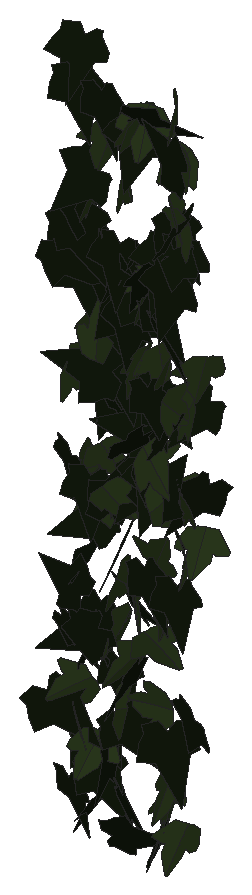
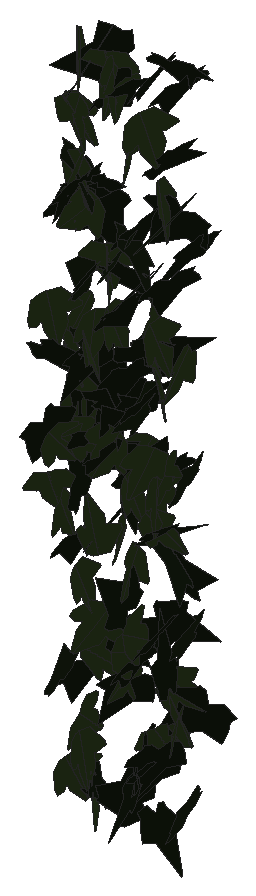
# SketchUp Ruby script. Lengths in inches.
U = 1.inch
M = Sketchup.active_model
def pt(a) = Geom::Point3d.new(a.map { |v| v * U })
def face(e, loops, mat)
  f = e.add_face(loops[0].map { |a| pt(a) })
  loops[1..].each { |l| e.add_face(l.map { |a| pt(a) }).erase! }
  f.material = f.back_material = mat if mat
  f
end
# faces: each face lists its corners as indices into pts; further lists are holes
def faces(e, pts, list, mat = nil) = list.each { |f| face(e, (f[0].is_a?(Array) ? f : [f]).map { |l| l.map { |i| pts[i] } }, mat) }
# xy, xz, yz: faces in a plane at the given z, y or x. An outline is a flat list of corners, or four numbers for a rectangle; further outlines are holes
def ring(l) = l.size == 4 ? [[l[0], l[1]], [l[2], l[1]], [l[2], l[3]], [l[0], l[3]]] : l.each_slice(2).to_a
def flat(e, list, mat, &to3) = list.each { |f| face(e, (f[0].is_a?(Array) ? f : [f]).map { |l| ring(l).map { |u, v| to3.(u, v) } }, mat) }
def xy(e, z, list, mat = nil) = flat(e, list, mat) { |x, y| [x, y, z] }
def xz(e, y, list, mat = nil) = flat(e, list, mat) { |x, z| [x, y, z] }
def yz(e, x, list, mat = nil) = flat(e, list, mat) { |y, z| [x, y, z] }
def lines(e, pts, list) = list.each { |a, b| e.add_line(pt(pts[a]), pt(pts[b])) }
# prism: a flat outline (further loops are holes) pulled along v
def prism(e, loops, v, mat = nil)
  f = face(e, loops, mat); d = Geom::Vector3d.new(v.map { |x| x * U })
  f.pushpull(f.normal.samedirection?(d) ? d.length : -d.length)
end
def box(e, o, s, mat = nil) = prism(e, [[o, [o[0] + s[0], o[1], o[2]], [o[0] + s[0], o[1] + s[1], o[2]], [o[0], o[1] + s[1], o[2]]]], [0, 0, s[2]], mat)
def at(x, y, z, deg = 0) = Geom::Transformation.translation(pt([x, y, z])) * Geom::Transformation.rotation(ORIGIN, Z_AXIS, deg.degrees)
def axes(o, x, y, z) = Geom::Transformation.new([*x, 0, *y, 0, *z, 0, *pt(o).to_a, 1])
def part(name) = M.definitions.add(name)
# library, detail: a bought-in or finely detailed component or shape, given as its bounding box
def library(name, o, s) = part(name).tap { |d| box(d.entities, o, s) }
def detail(e, o, s) = box(e.add_group.entities, o, s)
def put(e, d, t, mat = nil) = e.add_instance(d, t).tap { |i| i.material = mat if mat }
def group(e, t, mat = nil) = e.add_group.tap { |g| g.transformation = t; g.material = mat if mat }.entities
root = M.entities
M.materials.add("efeu1").color = [18, 25, 13]
M.materials.add("efeu2").color = [43, 57, 29]
c1 = part("ivyleaf_9")
p = [[1.54,2.16,1.25],[1.36,2.04,1.19],[-0.21,0.99,0.68],[-0.71,1.11,0.82],[-0.85,0.86,0.67],[-0.8,0.17,0.21],
  [-0.9,-0.01,0.1],[-0.67,-0.16,-0.02],[-0.08,-0.08,-0.05],[-0.03,-0.6,-0.4],[0.65,-0.88,-0.66],[0.83,-0.6,-0.49],
  [1.29,-0.42,-0.43],[1.8125,-0.07,-0.26],[1.21,0.44,0.15]]
faces(c1.entities,p,[[0,1,2,3,4,5,6,7,8,9,10,11,12,13,14]],"efeu1")
c2 = part("ivyleaf_10")
p = [[0,0.5,-0.03],[-0.0625,2.02,-0.43],[-0.19,2.01,-0.46],[-0.54,1.05,-0.29],[-0.52,0.625,-0.18],[-0.83,0.76,-0.28],
  [-1.16,0.64,-0.33],[-1.15,0.33,-0.24],[-0.77,-0.39,0.02],[-0.3,-0.51,0.16],[0.04,-0.48,0.23],[-0.02,2.01,-0.4375],
  [-0.06,2.01,-0.43],[0.04,-0.49,0.23],[0.67,-0.49,0.14],[1.38,0.36,-0.2],[1.375,0.51,-0.24],[0.81,0.65,-0.19],
  [0.62,0.59,-0.15],[0.6,1.09,-0.28],[0.5,1.23,-0.31]]
faces(c2.entities,p,[[0,1,2,3,4,5,6,7,8,9,10],[11,12,0,13,14,15,16,17,18,19,20]],"efeu2")
put(root,c1,axes([551.875,130.74,243.39],[-0.73548,-0.58268,-0.39107],[0.45946,0.02837,-0.90635],[0.53043,-0.8325,0.24283]))
put(root,c2,axes([551.63,130.18,211.08],[0.71363,-0.41325,-0.37001],[0.32522,-0.1767,0.82459],[-0.44935,-0.78419,0.00919]))
put(root,c1,axes([551.56,130.29,223.09],[0.17606,-0.69879,0.57439],[0.16825,-0.54966,-0.72027],[0.88877,0.24248,0.02257]))
put(root,c1,axes([551.46,128.98,212.17],[-0.08461,-0.32364,-1.03938],[0.63838,0.8297,-0.31032],[0.88178,-0.63173,0.12492]))
put(root,c1,axes([551.58,130.1875,207.4],[0.4557,-0.79853,0.24374],[0.10831,-0.21879,-0.9193],[0.82784,0.46819,-0.0139]))
put(root,c1,axes([551.75,129.03,234.1],[0.54072,-0.53779,-0.74074],[-0.22529,0.75567,-0.71309],[0.88722,0.51965,0.27038]))
put(root,c2,axes([552.82,129.55,212.97],[-0.44073,-0.23806,0.79955],[-0.61172,-0.52263,-0.49281],[0.56723,-0.74859,0.08978]))
put(root,c1,axes([551.875,129.42,215.66],[0.72537,-0.54547,-0.21984],[-0.11834,0.20656,-0.90298],[0.57608,0.72927,0.09133]))
put(root,c2,axes([552.93,130.6875,221.07],[-0.56763,0.02035,0.73262],[-0.65899,-0.41973,-0.49892],[0.32076,-0.8263,0.27148]))
put(root,c1,axes([552.2,130.6,213.66],[0.04903,0.69244,0.79719],[-0.13822,-0.78697,0.69207],[1.04684,-0.13634,0.05403]))
put(root,c1,axes([552.09,129.99,241.96],[0.10131,-0.9926,-0.20243],[0.02815,0.20612,-0.9966],[1.01264,0.09357,0.04796]))
put(root,c1,axes([553.18,128.72,217.72],[-0.19941,0.13422,0.89928],[-0.69386,0.57251,-0.23931],[-0.5876,-0.72159,-0.02259]))
put(root,c2,axes([552.375,130.49,223.46],[-0.04635,0.50692,-0.77285],[0.02045,-0.77307,-0.50829],[-0.92404,-0.04253,0.02752]))
put(root,c1,axes([552.99,129.21,218.8],[-0.20039,0.78529,0.56916],[-0.1994,0.53541,-0.80893],[-0.94914,-0.27828,0.04978]))
put(root,c2,axes([552.58,130.93,230.2],[0.06623,-0.95926,0.25328],[0.02269,-0.25231,-0.96153],[0.99187,0.06983,0.00508]))
put(root,c2,axes([552.44,129.15,228.34],[0.18841,-0.77312,-0.71532],[0.22398,0.73946,-0.74022],[1.02919,-0.0194,0.29204]))
put(root,c1,axes([552.24,130.46,232.69],[-0.04103,-0.92797,-0.29273],[0.03155,0.29157,-0.92871],[0.97254,-0.04861,0.01778]))
put(root,c2,axes([552.625,129.37,211.4],[-0.52676,0.73649,0.16397],[-0.11717,0.1177,-0.90509],[-0.74537,-0.53899,0.02641]))
put(root,c2,axes([552.61,130.81,228.21],[0.62375,-0.71751,-0.12292],[-0.04467,0.12384,-0.94956],[0.72659,0.62357,0.04714]))
put(root,c1,axes([552.95,130.4,206.96],[-0.39182,0.78825,-0.28221],[0.08901,-0.27061,-0.87941],[-0.83251,-0.39992,0.0388]))
put(root,c1,axes([552.98,130.84,220.37],[-0.65916,-0.26857,0.61132],[-0.35575,-0.58569,-0.64089],[0.56506,-0.68203,0.30963]))
put(root,c1,axes([552.19,129.89,235.78],[0.66785,-0.57956,-0.4415],[-0.13878,0.48676,-0.8489],[0.71523,0.63561,0.24754]))
put(root,c2,axes([552.81,130.49,222.6],[0.03199,-0.9257,-0.29655],[0.03115,0.29753,-0.92542],[0.97154,0.02094,0.03944]))
put(root,c2,axes([552.92,130.12,236.52],[0.37549,-0.93857,-0.20251],[-0.04385,0.20046,-1.01035],[0.95916,0.37659,0.03309]))
put(root,c1,axes([552.57,131.05,215.91],[0.20574,-0.92635,0.10949],[0.01826,-0.1081,-0.94891],[0.93262,0.20648,-0.00558]))
put(root,c1,axes([552.41,129.49,235.5],[-0.32673,-0.47618,-0.97385],[0.80772,0.57143,-0.55041],[0.723,-0.85358,0.17481]))
put(root,c1,axes([553.56,129.47,215.78],[-0.15472,-0.05646,-0.93104],[-0.37886,-0.8586,0.11503],[-0.85235,0.39189,0.11788]))
put(root,c1,axes([553.16,129.88,237.75],[-0.46724,-0.678,0.58718],[-0.2175,-0.55666,-0.81584],[0.87015,-0.5032,0.11137]))
put(root,c1,axes([552.96,130.32,209.98],[-0.04159,-0.76272,-0.61098],[-0.00593,0.61172,-0.76324],[0.97725,-0.02874,-0.03064]))
put(root,c2,axes([553.23,130.56,223.95],[-0.59059,-0.61552,-0.4088],[0.32802,0.25054,-0.85112],[0.66211,-0.67316,0.05702]))
put(root,c1,axes([553.15,131.18,226.97],[-0.14366,-0.92937,0.24009],[-0.0217,-0.23956,-0.94029],[0.95963,-0.14455,0.01468]))
put(root,c1,axes([554.01,129.77,228.35],[-0.52949,-0.5655,-0.666],[-0.2161,-0.66979,0.74053],[-0.84655,0.52468,0.22752]))
put(root,c2,axes([553.51,129.51,210.26],[0.6923,0.48876,-0.3775],[-0.29893,-0.23103,-0.84731],[-0.54041,0.75393,-0.01491]))
put(root,c2,axes([553.63,130.4375,239.68],[-0.45807,-0.87367,0.30003],[-0.05476,-0.30863,-0.98229],[0.92213,-0.45232,0.09071]))
put(root,c1,axes([553.6,131.15,229.36],[-0.66621,-0.65807,0.06911],[-0.04349,-0.05431,-0.93639],[0.66025,-0.66758,0.00805]))
put(root,c1,axes([553.26,129.51,222.96],[-0.08448,-0.91933,-0.11123],[-0.00032,0.11172,-0.92315],[0.92604,-0.08383,-0.01046]))
put(root,c1,axes([553.28,129.9375,209],[0.16461,-0.78141,-0.53609],[-0.01765,0.54149,-0.7947],[0.94746,0.14585,0.07834]))
put(root,c1,axes([553.11,130.89,226.72],[0.71599,-0.66448,0.00847],[0.00634,-0.00562,-0.97682],[0.66451,0.71602,0.0002]))
put(root,c2,axes([553.9,130.97,222.57],[0.16534,-0.90004,0.23776],[0.04672,-0.23316,-0.9151],[0.92974,0.17178,0.0037]))
put(root,c2,axes([554.07,128.74,229.93],[0.06984,0.83129,-0.62397],[-0.08929,0.62786,0.82649],[1.03558,-0.00193,0.11334]))
put(root,c2,axes([553.76,131.11,215.55],[0.19819,-0.45252,0.84638],[0.33029,-0.77929,-0.49399],[0.90114,0.38516,-0.00509]))
put(root,c1,axes([553.64,129.77,241.71],[0.2977,-0.95907,-0.03031],[-0.00381,0.03056,-1.0042],[0.95954,0.29768,0.00542]))
put(root,c1,axes([553.84,130.17,209.64],[-0.06147,0.02149,-0.92568],[0.73848,-0.5585,-0.06201],[-0.55856,-0.74077,0.0199]))
put(root,c1,axes([554.82,129.71,233.39],[-0.44739,0.86442,0.32225],[-0.14569,0.28745,-0.97333],[-0.91096,-0.47051,-0.0026]))
put(root,c1,axes([554.15,130.32,231.23],[-0.20226,-0.61899,0.74105],[-0.01088,-0.75562,-0.63414],[0.9655,-0.13819,0.14809]))
put(root,c1,axes([554.13,130.92,228.01],[-0.03933,-0.90661,-0.33703],[0.00879,0.33696,-0.90745],[0.96719,-0.03993,-0.00546]))
put(root,c1,axes([554.13,130.39,213.89],[0.17353,-0.85237,-0.15761],[-0.03683,0.15334,-0.86984],[0.86603,0.17731,-0.00541]))
put(root,c1,axes([554.3125,130.14,207.82],[0.72436,-0.2885,-0.50061],[-0.46209,0.19267,-0.77967],[0.34686,0.85918,0.00675]))
put(root,c2,axes([554.59,129.72,218.41],[0.02497,-0.64407,-0.77364],[-0.02369,0.77329,-0.64454],[1.00637,0.03419,0.00403]))
put(root,c1,axes([554.32,130.1,234.36],[-0.04651,-0.98064,0.04025],[-0.00607,-0.04,-0.98174],[0.98145,-0.04672,-0.00417]))
put(root,c2,axes([554.61,130.67,214.28],[0.01996,-0.34084,0.87208],[0.10066,-0.86645,-0.34094],[0.9309,0.10099,0.01817]))
put(root,c1,axes([554.48,131.08,230.83],[-0.12764,-0.95999,0.10839],[-0.01143,-0.10782,-0.96843],[0.96602,-0.12812,0.00286]))
put(root,c1,axes([554.01,131.13,216.79],[0.3423,-0.47171,0.80009],[0.52691,-0.60357,-0.58128],[0.76486,0.62691,0.04237]))
put(root,c1,axes([554.6875,129.11,222.15],[-0.40003,-0.30044,0.87943],[0.67287,0.56677,0.4997],[-0.64102,0.78242,-0.02428]))
put(root,c1,axes([555.21,130.44,232.18],[-0.92665,-0.19236,0.12728],[-0.12159,-0.04043,-0.94629],[0.19601,-0.93448,0.01474]))
put(root,c1,axes([554.4375,131.04,233.45],[0.43378,-0.86158,0.16841],[0.06689,-0.15486,-0.96457],[0.87534,0.4388,-0.00975]))
put(root,c2,axes([555.03,129.51,238.23],[0.40796,-0.76983,-0.51925],[0.01721,0.57333,-0.83648],[0.92842,0.32765,0.24368]))
put(root,c1,axes([554.63,130.41,231.01],[0.02632,-0.91806,0.3378],[0.09384,-0.33399,-0.91502],[0.97372,0.05701,0.07905]))
put(root,c2,axes([554.83,128.77,223.17],[-0.55275,-0.54128,-0.53516],[0.43401,0.3192,-0.77114],[0.62531,-0.70003,0.06216]))
put(root,c1,axes([555.88,130.5,225.73],[-0.57471,0.20172,0.72488],[-0.75187,-0.18893,-0.54353],[0.02884,-0.90556,0.27487]))
put(root,c2,axes([555.18,129.11,212.65],[0.1565,-0.37876,-0.92256],[0.15558,0.93169,-0.35611],[0.98507,-0.08698,0.20281]))
put(root,c1,axes([555.32,129.42,221.09],[-0.50416,0.11978,-0.79649],[0.64666,-0.49999,-0.48452],[-0.48018,-0.79911,0.18376]))
put(root,c1,axes([555.5,130.86,223.37],[-0.49577,-0.73784,0.29071],[-0.17972,-0.22939,-0.8887],[0.77241,-0.52695,-0.02019]))
put(root,c2,axes([555.21,130.59,224.11],[-0.9553,0.2278,-0.36849],[0.35812,-0.0868,-0.98209],[-0.24378,-1.02022,0.00128]))
put(root,c1,axes([555.55,129.73,214.46],[-0.43371,0.30992,-0.7181],[0.45152,-0.57126,-0.51925],[-0.63863,-0.61437,0.12057]))
put(root,c1,axes([555.2,129.31,212.15],[-0.06442,-0.53687,-0.74799],[0.11812,0.73881,-0.54045],[0.91311,-0.13345,0.01714]))
put(root,c2,axes([555.61,130.02,229.55],[0.19529,-0.97298,0.24226],[0.04322,-0.23841,-0.99237],[1.00175,0.19997,-0.00441]))
put(root,c2,axes([555.43,130.55,233.07],[0.88497,0.37488,-0.01986],[-0.01846,-0.00735,-0.9611],[-0.37496,0.88516,0.00043]))
put(root,c2,axes([555.72,129.74,241.05],[-0.05998,-0.99727,-0.13968],[0.02913,0.13815,-0.99886],[1.00658,-0.06342,0.02058]))
put(root,c1,axes([555.45,130.1875,240.39],[-0.30176,-0.95655,0.15088],[0.0368,-0.16924,-0.99941],[0.96768,-0.29185,0.08505]))
put(root,c2,axes([555.73,130.1,232.58],[0.36943,-0.81428,-0.38138],[-0.04982,0.39315,-0.88766],[0.89779,0.35689,0.10768]))
put(root,c1,axes([554.9375,129.06,206.36],[0.465,-0.05133,0.75556],[0.75284,-0.06475,-0.46773],[0.08207,0.88482,0.0096]))
put(root,c2,axes([555.79,129.61,241.18],[-0.03077,-0.88523,-0.54951],[0.04613,0.54805,-0.88546],[1.04089,-0.05046,0.023]))
put(root,c1,axes([555.84,128.79,226.05],[0.3555,0.85856,0.21497],[0.09497,0.19332,-0.92916],[-0.87996,0.36773,-0.01343]))
put(root,c2,axes([555.74,130.56,215.59],[-0.7126,-0.42287,-0.54351],[0.48497,0.24712,-0.82811],[0.48891,-0.86148,0.02925]))
put(root,c2,axes([555.76,130.84,219.23],[-0.88094,-0.05765,0.45851],[0.46154,-0.0604,0.87917],[-0.02311,0.99128,0.08024]))
put(root,c2,axes([555.92,129.05,218.8],[-0.45193,0.77193,-0.35043],[0.15694,-0.31406,-0.89423],[-0.83309,-0.47792,0.02164]))
put(root,c2,axes([556.05,130.66,229.5625],[-0.24647,-0.9224,-0.17623],[0.21307,0.12251,-0.93926],[0.91459,-0.27711,0.17133]))
put(root,c2,axes([556.14,129.63,241.55],[0.96341,0.33112,-0.07589],[-0.07657,-0.01067,-1.01862],[-0.33096,0.96633,0.01475]))
put(root,c2,axes([556.24,130.85,228.81],[0.45979,-0.85197,0.10793],[0.05793,-0.09138,-0.96809],[0.85683,0.46336,0.00753]))
put(root,c2,axes([557.04,129.58,213.1],[0.18421,-0.06106,-0.98342],[-0.94164,0.28364,-0.19399],[0.29009,0.95947,-0.00524]))
put(root,c2,axes([556.52,131.03,217.46],[0.16967,-0.8968,0.20543],[0.00988,-0.20711,-0.91228],[0.91998,0.16762,-0.02809]))
put(root,c1,axes([556.47,130.32,224],[-0.47462,-0.86682,0.00865],[-0.00326,-0.00807,-0.98825],[0.86686,-0.47463,0.00102]))
put(root,c1,axes([556.13,130.31,232.15],[0.48133,-0.83711,-0.26429],[-0.07022,0.26373,-0.96322],[0.87502,0.48164,0.06808]))
put(root,c1,axes([556.88,129.29,234.58],[-0.12748,0.82066,-0.53662],[0.07038,-0.53208,-0.83044],[-0.978,-0.14526,0.01019]))
put(root,c2,axes([556.81,129.8125,206.93],[0.31844,-0.72157,-0.55667],[-0.21518,0.51347,-0.78867],[0.88557,0.38423,0.00854]))
put(root,c1,axes([556.16,129.59,219.46],[0.41966,-0.9137,-0.14989],[-0.06587,0.13469,-1.00546],[0.92357,0.42479,-0.0036]))
put(root,c1,axes([555.89,129.23,241.5],[0.80072,-0.06343,0.62804],[0.63109,0.10206,-0.7943],[-0.01345,1.01251,0.1194]))
put(root,c2,axes([557.37,130.08,223.54],[-0.30567,-0.01907,0.86678],[-0.8361,-0.23667,-0.30006],[0.22937,-0.88811,0.06135]))
put(root,c1,axes([556.4,129.52,228.37],[0.30368,-0.88911,-0.13461],[-0.03353,0.13079,-0.93948],[0.89862,0.30534,0.01044]))
put(root,c1,axes([556.56,130.18,227.73],[0.13753,-0.6209,-0.70327],[-0.15716,0.68549,-0.63594],[0.92488,0.20881,-0.00349]))
put(root,c2,axes([556.39,130.66,235.03],[-0.76359,0.05736,-0.64789],[0.63893,-0.12087,-0.76373],[-0.12175,-0.99409,0.05548]))
put(root,c2,axes([557.27,130.71,239.49],[0.81678,-0.08133,-0.53812],[-0.52615,0.13009,-0.81826],[0.13913,0.96942,0.06467]))
put(root,c2,axes([556.9375,130.57,236.97],[-0.47893,0.85947,-0.04097],[0.04225,-0.02334,-0.98357],[-0.85941,-0.48012,-0.02552]))
put(root,c2,axes([557.125,130.13,208.85],[0.05689,-0.98371,-0.05333],[0.00026,0.05344,-0.98534],[0.98515,0.05679,0.00334]))
put(root,c2,axes([557.34,130.55,239.48],[0.69738,-0.36658,-0.58266],[-0.40167,0.45689,-0.7682],[0.55905,0.78555,0.1749]))
put(root,c1,axes([556.71,130.86,236.07],[0.31154,-0.85778,-0.38902],[-0.08652,0.38195,-0.91149],[0.93789,0.32016,0.04514]))
put(root,c1,axes([557.38,128.625,206.5],[0.02013,0.3719,0.82199],[-0.0515,0.82133,-0.37034],[-0.90074,-0.03865,0.03954]))
put(root,c1,axes([557.65,129.59,236.21],[-0.24875,0.83909,0.45306],[-0.22015,0.40504,-0.87103],[-0.92783,-0.32107,0.0852]))
put(root,c2,axes([557.59,130.25,236.35],[0.67278,-0.2848,-0.69572],[-0.5409,0.46501,-0.71342],[0.52208,0.84878,0.15741]))
put(root,c1,axes([556.68,130.83,221.25],[0.1809,-0.37712,0.89341],[0.32776,-0.83156,-0.41738],[0.91268,0.37338,-0.02719]))
put(root,c2,axes([557.1,128.7,225.64],[0.11098,0.99056,0.40153],[0.05037,0.3984,-0.99674],[-1.06766,0.12176,-0.00528]))
put(root,c1,axes([556.9,129.19,223.12],[-0.5442,0.19753,0.8737],[0.75806,-0.44306,0.57234],[0.4772,0.92909,0.08718]))
put(root,c2,axes([557.45,129.95,242.18],[0.46237,-0.78657,-0.53416],[-0.12012,0.54089,-0.90045],[0.94318,0.45448,0.14718]))
put(root,c1,axes([557.33,129.91,235.25],[-0.59329,-0.79156,-0.13412],[0.06581,0.11825,-0.98906],[0.80014,-0.59666,-0.0181]))
put(root,c2,axes([557.52,131.01,220.39],[-0.26781,0.80978,-0.32486],[-0.21537,-0.39066,-0.79624],[-0.84551,-0.15698,0.30572]))
put(root,c2,axes([557.26,128.98,223.28],[0.1853,0.16928,-0.99561],[0.32913,0.94685,0.22224],[0.95476,-0.35926,0.11662]))
put(root,c1,axes([557.27,130.625,235.01],[-0.26045,-0.94381,-0.16763],[0.03014,0.16556,-0.97897],[0.9581,-0.26177,-0.01477]))
put(root,c2,axes([557.56,129.59,209.79],[0.03164,0.72627,-0.77199],[-0.08628,-0.768,-0.72605],[-1.0564,0.08448,0.03617]))
put(root,c1,axes([556.96,129.77,231.18],[0.4857,-0.7106,0.56644],[0.30014,-0.48079,-0.8605],[0.85774,0.57061,-0.01965]))
put(root,c1,axes([558.18,128.58,227.21],[-0.38231,0.79811,0.36598],[-0.20969,0.30462,-0.88335],[-0.85261,-0.43279,0.05315]))
put(root,c1,axes([557.39,130.18,218.71],[0.05479,-0.92556,-0.13576],[-0.03282,0.13401,-0.92686],[0.93489,0.05895,-0.02458]))
put(root,c1,axes([558.03,129.52,239.61],[0.12959,-1.02922,0.25517],[0.02242,0.25967,1.03598],[-1.06014,-0.12032,0.0531]))
put(root,c2,axes([557.87,131.01,223.47],[-0.24363,-0.63617,0.61967],[0.10867,-0.65909,-0.63391],[0.88141,-0.09458,0.24944]))
put(root,c2,axes([558.05,130.04,227.83],[0.80966,-0.62266,-0.31627],[-0.25314,0.18963,-1.02139],[0.65088,0.8483,-0.00381]))
put(root,c1,axes([557.68,129.65,234.08],[-0.1638,-0.97246,0.28858],[0.00288,-0.29276,-0.98492],[1.01437,-0.1562,0.04939]))
put(root,c2,axes([558.07,129.76,207.27],[-0.33665,-0.78974,0.45111],[0.03524,-0.49199,-0.835],[0.90882,-0.27347,0.19948]))
put(root,c1,axes([557.66,129.26,212.14],[0.06106,-1.03723,-0.32249],[-0.02678,0.32146,-1.039],[1.08587,0.06625,-0.00749]))
put(root,c1,axes([558.33,131.13,227.74],[-0.88742,-0.28168,0.01555],[-0.0153,-0.00322,-0.93105],[0.2817,-0.88755,-0.00156]))
put(root,c1,axes([557.71,130.9,212.11],[-0.00968,-0.61314,0.74194],[0.21352,-0.72486,-0.59624],[0.93852,0.15859,0.1433]))
put(root,c2,axes([558.36,130.81,229.7],[-0.45957,-0.84302,0.16484],[-0.04532,-0.1629,-0.95941],[0.85779,-0.46026,0.03763]))
put(root,c2,axes([558.35,128.47,228.68],[-0.06551,0.64096,0.71049],[-0.23443,0.6797,-0.6348],[-0.92772,-0.21702,0.11024]))
put(root,c2,axes([558.65,129.01,224.03],[-0.72856,0.42313,0.49402],[-0.43269,0.23858,-0.84247],[-0.48566,-0.84731,0.00948]))
put(root,c2,axes([558.32,130.74,221.31],[0.73398,0.52199,-0.18628],[-0.13513,-0.13124,-0.90023],[-0.53751,0.74579,-0.02804]))
put(root,c1,axes([558.58,130.78,223.86],[-0.04249,0.29166,-0.91526],[0.12545,-0.90662,-0.29473],[-0.95238,-0.13243,0.00202]))
